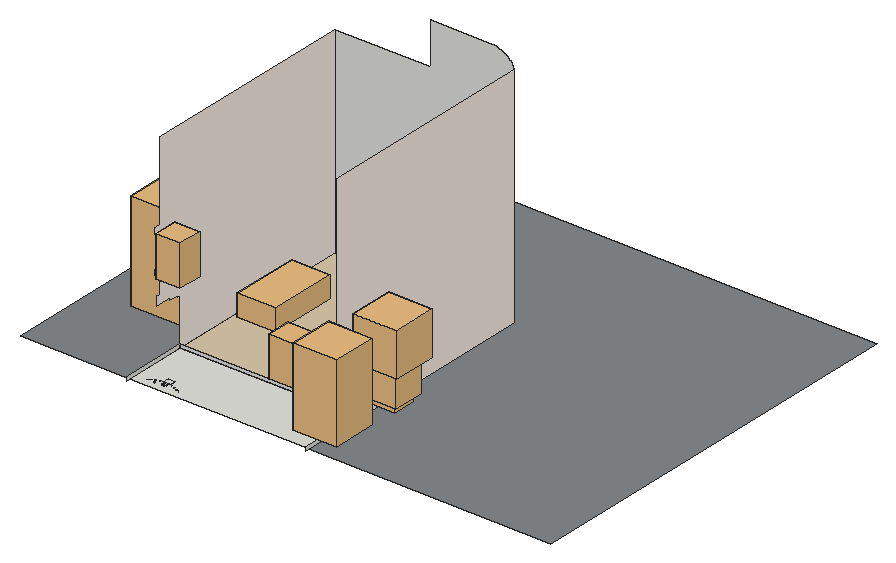
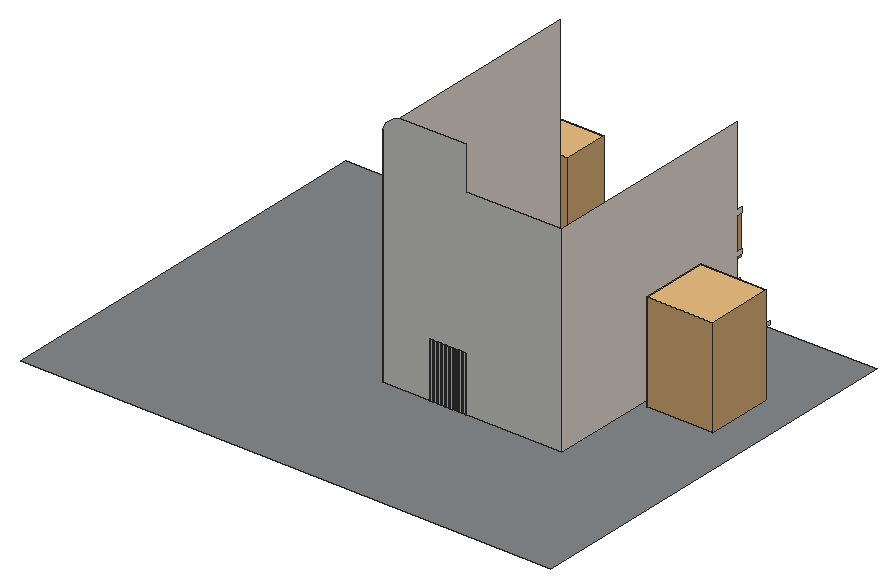
# SketchUp Ruby script. Lengths in inches.
U = 1.inch
M = Sketchup.active_model
def pt(a) = Geom::Point3d.new(a.map { |v| v * U })
def face(e, loops, mat)
  f = e.add_face(loops[0].map { |a| pt(a) })
  loops[1..].each { |l| e.add_face(l.map { |a| pt(a) }).erase! }
  f.material = f.back_material = mat if mat
  f
end
# faces: each face lists its corners as indices into pts; further lists are holes
def faces(e, pts, list, mat = nil) = list.each { |f| face(e, (f[0].is_a?(Array) ? f : [f]).map { |l| l.map { |i| pts[i] } }, mat) }
# xy, xz, yz: faces in a plane at the given z, y or x. An outline is a flat list of corners, or four numbers for a rectangle; further outlines are holes
def ring(l) = l.size == 4 ? [[l[0], l[1]], [l[2], l[1]], [l[2], l[3]], [l[0], l[3]]] : l.each_slice(2).to_a
def flat(e, list, mat, &to3) = list.each { |f| face(e, (f[0].is_a?(Array) ? f : [f]).map { |l| ring(l).map { |u, v| to3.(u, v) } }, mat) }
def xy(e, z, list, mat = nil) = flat(e, list, mat) { |x, y| [x, y, z] }
def xz(e, y, list, mat = nil) = flat(e, list, mat) { |x, z| [x, y, z] }
def yz(e, x, list, mat = nil) = flat(e, list, mat) { |y, z| [x, y, z] }
def lines(e, pts, list) = list.each { |a, b| e.add_line(pt(pts[a]), pt(pts[b])) }
# prism: a flat outline (further loops are holes) pulled along v
def prism(e, loops, v, mat = nil)
  f = face(e, loops, mat); d = Geom::Vector3d.new(v.map { |x| x * U })
  f.pushpull(f.normal.samedirection?(d) ? d.length : -d.length)
end
def box(e, o, s, mat = nil) = prism(e, [[o, [o[0] + s[0], o[1], o[2]], [o[0] + s[0], o[1] + s[1], o[2]], [o[0], o[1] + s[1], o[2]]]], [0, 0, s[2]], mat)
def at(x, y, z, deg = 0) = Geom::Transformation.translation(pt([x, y, z])) * Geom::Transformation.rotation(ORIGIN, Z_AXIS, deg.degrees)
def axes(o, x, y, z) = Geom::Transformation.new([*x, 0, *y, 0, *z, 0, *pt(o).to_a, 1])
def part(name) = M.definitions.add(name)
# library, detail: a bought-in or finely detailed component or shape, given as its bounding box
def library(name, o, s) = part(name).tap { |d| box(d.entities, o, s) }
def detail(e, o, s) = box(e.add_group.entities, o, s)
def put(e, d, t, mat = nil) = e.add_instance(d, t).tap { |i| i.material = mat if mat }
def group(e, t, mat = nil) = e.add_group.tap { |g| g.transformation = t; g.material = mat if mat }.entities
root = M.entities
M.materials.add("Material__3").color = [91, 133, 74]
M.materials.add("Material__4").color = [174, 125, 66]
M.materials.add("[0009_Linen]").color = [250, 240, 230]
M.materials.add("[Asphalt_Stamped_Brick]").color = [149, 133, 134]
M.materials.add("[Blacktop Old 01]").color = [132, 136, 139]
M.materials.add("[Brick_Colored_Blue]").color = [144, 143, 146]
M.materials.add("[Field Square Tile]").color = [217, 201, 169]
M.materials.add("[Metal_Steel_Textured_White]").color = [191, 191, 191]
c1 = library("Group\#1",[-35.09,50.53,0.35],[65,65.01,78.63])
c2 = library("Group\#5",[-64.15,18.03,113.23],[126.13,128.06,125.3])
c3 = library("Group\#6",[-43.12,34.07,23.92],[89.16,89.66,208.68])
c4 = library("Group\#120",[0,0,0],[26.57,25.63,42.93])
c5 = library("Group\#10",[-45.81,-5.78,22.29],[23.07,17.06,86])
c6 = library("Group\#3",[0,0,0],[46.67,47.38,83.02])
c7 = part("BAMBOO+PLANTS+18")
p = [[0,0,0],[1,0,0],[1,1,0]]
lines(c7.entities,p,[[0,1],[1,2],[2,0]])
put(c7.entities,c1,at(0,0,0))
put(c7.entities,c2,at(0,0,0),"Material__3")
put(c7.entities,c3,at(0,0,0),"Material__4")
put(c7.entities,c4,axes([-354.27,77.73,-57.76],[2.7027,0,0],[0,2.7027,0],[0,0,2.7027]))
put(c7.entities,c4,axes([-609.51,-13.32,151.65],[2.7027,0,0],[0,2.7027,0],[0,0,2.7027]))
put(c7.entities,c5,at(0,0,0),"Material__4")
put(c7.entities,c6,axes([-100.4,-152.87,0.24],[2.7027,0,0],[0,2.7027,0],[0,0,2.7027]))
put(c7.entities,c6,axes([-818.61,158.75,-120.63],[4.05405,0,0],[0,4.05405,0],[0,0,4.05405]))
c8 = library("office",[0,0,0],[107.02,69.62,36.57])
c9 = part("Vertical timber slat")
box(c9.entities,[0,0,0],[1.85,1.85,112.2])
c10 = part("Timber slat screen")
put(c10.entities,c9,at(0,0,0))
put(c10.entities,c9,at(0,13.1875,0))
put(c10.entities,c9,at(0,18.46,0))
put(c10.entities,c9,at(0,10.55,0))
put(c10.entities,c9,at(0,2.64,0))
put(c10.entities,c9,at(0,7.91,0))
put(c10.entities,c9,at(0,5.28,0))
put(c10.entities,c9,at(0,15.83,0))
put(c10.entities,c9,at(0,21.1,0))
xy(root,0,[[116.615,181.5,303.95,249.09],[303.95,181.5,308.325,249.09]])
xy(root,0,[[0,181.5,0,616,566.5625,616,566.5625,181.5,308.325,181.5,308.325,455.527,116.615,455.527,116.615,181.5]],"[Blacktop Old 01]")
xy(root,0,[[116.615,249.09,308.325,455.527]],"[Field Square Tile]")
xy(root,3.625,[[141.398,184.727,141.393,184.728,141.388,184.73,141.384,184.733,141.381,184.737,141.379,184.742,141.378,184.747,141.379,184.752,141.381,184.757,141.384,184.761,141.388,184.765,141.393,184.767,141.404,184.767,141.408,184.765,141.416,184.757,141.418,184.752,141.418,184.742,141.416,184.737,141.412,184.733,141.408,184.73,141.404,184.728],[148.82,185.161,148.815,185.162,148.81,185.164,148.806,185.167,148.803,185.171,148.801,185.176,148.8,185.181,148.801,185.187,148.803,185.191,148.806,185.196,148.81,185.199,148.815,185.201,148.825,185.201,148.83,185.199,148.834,185.196,148.837,185.191,148.839,185.187,148.84,185.181,148.839,185.176,148.837,185.171,148.834,185.167,148.83,185.164,148.825,185.162],[150.816,185.161,150.811,185.162,150.806,185.164,150.802,185.167,150.799,185.171,150.797,185.176,150.796,185.181,150.797,185.187,150.799,185.191,150.802,185.196,150.806,185.199,150.811,185.201,150.821,185.201,150.826,185.199,150.83,185.196,150.833,185.191,150.835,185.187,150.836,185.181,150.835,185.176,150.833,185.171,150.83,185.167,150.826,185.164,150.821,185.162],[163.155,185.926,163.15,185.927,163.145,185.929,163.141,185.932,163.138,185.936,163.136,185.941,163.135,185.946,163.136,185.951,163.138,185.956,163.141,185.96,163.145,185.964,163.15,185.966,163.161,185.966,163.165,185.964,163.173,185.956,163.175,185.951,163.175,185.941,163.173,185.936,163.169,185.932,163.165,185.929,163.161,185.927],[147.357,186.909,147.351,186.91,147.347,186.912,147.343,186.915,147.339,186.919,147.337,186.924,147.337,186.934,147.339,186.939,147.343,186.943,147.347,186.946,147.351,186.948,147.357,186.949,147.362,186.948,147.367,186.946,147.371,186.943,147.374,186.939,147.376,186.934,147.377,186.929,147.376,186.924,147.374,186.919,147.371,186.915,147.367,186.912,147.362,186.91],
  [152.279,186.909,152.274,186.91,152.269,186.912,152.265,186.915,152.262,186.919,152.26,186.924,152.259,186.929,152.26,186.934,152.262,186.939,152.265,186.943,152.269,186.946,152.274,186.948,152.279,186.949,152.284,186.948,152.289,186.946,152.293,186.943,152.296,186.939,152.298,186.934,152.299,186.929,152.298,186.924,152.296,186.919,152.293,186.915,152.289,186.912,152.284,186.91],[139.413,187.422,139.408,187.424,139.404,187.428,139.401,187.432,139.399,187.436,139.398,187.442,139.399,187.447,139.401,187.452,139.404,187.456,139.408,187.459,139.413,187.461,139.418,187.462,139.423,187.461,139.428,187.459,139.432,187.456,139.435,187.452,139.4375,187.447,139.438,187.442,139.4375,187.436,139.435,187.432,139.432,187.428,139.428,187.424,139.423,187.422],[140.156,187.727,140.151,187.728,140.146,187.73,140.142,187.733,140.138,187.737,140.136,187.742,140.136,187.752,140.138,187.757,140.142,187.761,140.146,187.764,140.151,187.766,140.156,187.767,140.161,187.766,140.166,187.764,140.17,187.761,140.173,187.757,140.175,187.752,140.176,187.747,140.175,187.742,140.173,187.737,140.17,187.733,140.166,187.73,140.161,187.728],[159.48,187.727,159.475,187.728,159.47,187.73,159.466,187.733,159.463,187.737,159.461,187.742,159.46,187.747,159.461,187.752,159.463,187.757,159.466,187.761,159.47,187.764,159.475,187.766,159.48,187.767,159.485,187.766,159.49,187.764,159.494,187.761,159.497,187.757,159.499,187.752,159.5,187.747,159.499,187.742,159.497,187.737,159.494,187.733,159.49,187.73,159.485,187.728],[156.044,188.822,156.039,188.824,156.035,188.827,156.032,188.831,156.03,188.836,156.029,188.841,156.03,188.847,156.032,188.851,156.035,188.856,156.039,188.859,156.044,188.861,156.054,188.861,156.059,188.859,156.063,188.856,156.066,188.851,156.068,188.847,156.069,188.841,156.068,188.836,156.066,188.831,156.063,188.827,156.059,188.824,156.054,188.822],
  [147.136,189.435,147.13,189.436,147.126,189.438,147.122,189.441,147.118,189.445,147.116,189.45,147.116,189.46,147.118,189.465,147.122,189.469,147.126,189.472,147.13,189.474,147.136,189.475,147.141,189.474,147.146,189.472,147.15,189.469,147.153,189.465,147.155,189.46,147.156,189.455,147.155,189.45,147.153,189.445,147.15,189.441,147.146,189.438,147.141,189.436],[148.537,189.542,148.532,189.544,148.528,189.548,148.525,189.552,148.523,189.557,148.522,189.562,148.523,189.567,148.525,189.572,148.528,189.576,148.532,189.579,148.537,189.581,148.542,189.582,148.547,189.581,148.552,189.579,148.556,189.576,148.56,189.572,148.562,189.567,148.562,189.557,148.56,189.552,148.552,189.544,148.547,189.542],[151.088,189.542,151.084,189.544,151.079,189.548,151.076,189.552,151.074,189.557,151.074,189.567,151.076,189.572,151.079,189.576,151.084,189.579,151.088,189.581,151.094,189.582,151.099,189.581,151.103,189.579,151.108,189.576,151.111,189.572,151.113,189.567,151.113,189.557,151.111,189.552,151.108,189.548,151.103,189.544,151.099,189.542]],"[Asphalt_Stamped_Brick]")
xy(root,3.625,[[148.272,184.789,148.267,184.793,148.262,184.796,148.258,184.799,148.238,184.811,148.233,184.815,148.234,184.82,148.234,184.832,148.235,184.838,148.235,184.849,148.236,184.855,148.236,184.861,148.241,184.863,148.246,184.866,148.251,184.868,148.256,184.871,148.262,184.874,148.267,184.876,148.272,184.879,148.277,184.881,148.292,184.872,148.296,184.869,148.306,184.863,148.311,184.859,148.316,184.856,148.315,184.85,148.315,184.839,148.314,184.833,148.314,184.822,148.313,184.816,148.313,184.81,148.308,184.808,148.298,184.802,148.293,184.8,148.287,184.797,148.282,184.795]],"[Brick_Colored_Blue]")
xy(root,3.625,[[[140.661,184.353,140.638,184.356,140.616,184.365,140.598,184.379,140.584,184.397,140.575,184.419,140.572,184.442,140.575,184.465,140.584,184.486,140.598,184.505,140.616,184.519,140.638,184.528,140.661,184.531,140.684,184.528,140.705,184.519,140.724,184.505,140.738,184.486,140.747,184.465,140.75,184.442,140.747,184.419,140.738,184.397,140.724,184.379,140.705,184.365,140.684,184.356],[140.661,184.354,140.683,184.357,140.705,184.366,140.723,184.38,140.737,184.398,140.746,184.419,140.749,184.442,140.746,184.464,140.737,184.486,140.723,184.504,140.705,184.518,140.683,184.527,140.661,184.53,140.638,184.527,140.617,184.518,140.599,184.504,140.585,184.486,140.576,184.464,140.573,184.442,140.576,184.419,140.585,184.398,140.599,184.38,140.617,184.366,140.638,184.357]],[[140.661,184.354,140.638,184.357,140.617,184.366,140.599,184.38,140.585,184.398,140.576,184.419,140.573,184.442,140.576,184.464,140.585,184.486,140.599,184.504,140.617,184.518,140.638,184.527,140.661,184.53,140.683,184.527,140.705,184.518,140.723,184.504,140.737,184.486,140.746,184.464,140.749,184.442,140.746,184.419,140.737,184.398,140.723,184.38,140.705,184.366,140.683,184.357],[140.661,184.405,140.67,184.406,140.679,184.41,140.687,184.416,140.692,184.423,140.696,184.432,140.697,184.442,140.696,184.451,140.692,184.46,140.687,184.468,140.679,184.473,140.67,184.477,140.661,184.478,140.651,184.477,140.642,184.473,140.635,184.468,140.629,184.46,140.625,184.451,140.624,184.442,140.625,184.432,140.629,184.423,140.635,184.416,140.642,184.41,140.651,184.406]],[[141.398,184.658,141.375,184.661,141.354,184.67,141.335,184.684,141.321,184.703,141.3125,184.724,141.309,184.747,141.3125,184.77,141.321,184.792,141.335,184.81,141.354,184.824,141.375,184.833,141.398,184.836,141.421,184.833,141.443,184.824,141.461,184.81,141.475,184.792,141.484,184.77,141.487,184.747,141.484,184.724,141.475,184.703,141.461,184.684,141.443,184.67,141.421,184.661],[141.398,184.659,141.421,184.662,141.442,184.671,141.461,184.685,141.474,184.703,141.483,184.724,141.486,184.747,141.483,184.77,141.474,184.791,141.461,184.809,141.442,184.823,141.421,184.832,141.398,184.835,141.376,184.832,141.354,184.823,141.336,184.809,141.322,184.791,141.313,184.77,141.31,184.747,141.313,184.724,141.322,184.703,141.336,184.685,141.354,184.671,141.376,184.662]],[[158.237,184.659,158.215,184.662,158.193,184.671,158.175,184.685,158.161,184.703,158.153,184.724,158.15,184.747,158.153,184.77,158.161,184.791,158.175,184.809,158.193,184.823,158.215,184.832,158.237,184.835,158.26,184.832,158.281,184.823,158.3,184.809,158.314,184.791,158.322,184.77,158.325,184.747,158.322,184.724,158.314,184.703,158.3,184.685,158.281,184.671,158.26,184.662],[158.237,184.711,158.247,184.712,158.256,184.716,158.263,184.721,158.269,184.729,158.273,184.738,158.274,184.747,158.273,184.757,158.269,184.766,158.263,184.773,158.256,184.779,158.247,184.783,158.237,184.784,158.228,184.783,158.219,184.779,158.212,184.773,158.206,184.766,158.202,184.757,158.201,184.747,158.202,184.738,158.206,184.729,158.212,184.721,158.219,184.716,158.228,184.712]],[[148.275,184.669,148.231,184.675,148.191,184.691,148.157,184.718,148.13,184.752,148.114,184.792,148.108,184.835,148.114,184.878,148.13,184.919,148.157,184.953,148.191,184.979,148.231,184.996,148.275,185.002,148.318,184.996,148.358,184.979,148.392,184.953,148.419,184.919,148.435,184.878,148.441,184.835,148.435,184.792,148.419,184.752,148.392,184.718,148.358,184.691,148.318,184.675],[148.275,184.716,148.306,184.72,148.334,184.732,148.359,184.751,148.378,184.776,148.39,184.804,148.394,184.835,148.39,184.866,148.378,184.895,148.359,184.92,148.334,184.939,148.306,184.951,148.275,184.955,148.244,184.951,148.215,184.939,148.19,184.92,148.171,184.895,148.159,184.866,148.155,184.835,148.159,184.804,148.171,184.776,148.19,184.751,148.215,184.732,148.244,184.72]],
  [[141.398,184.711,141.389,184.712,141.38,184.716,141.372,184.721,141.367,184.729,141.363,184.738,141.362,184.747,141.363,184.757,141.367,184.766,141.372,184.773,141.38,184.779,141.389,184.783,141.398,184.784,141.408,184.783,141.417,184.779,141.424,184.773,141.43,184.766,141.434,184.757,141.435,184.747,141.434,184.738,141.43,184.729,141.424,184.721,141.417,184.716,141.408,184.712],[141.398,184.727,141.404,184.728,141.408,184.73,141.412,184.733,141.416,184.737,141.418,184.742,141.418,184.752,141.416,184.757,141.408,184.765,141.404,184.767,141.393,184.767,141.388,184.765,141.384,184.761,141.381,184.757,141.379,184.752,141.378,184.747,141.379,184.742,141.381,184.737,141.384,184.733,141.388,184.73,141.393,184.728]],[[148.275,184.716,148.244,184.72,148.215,184.732,148.19,184.751,148.171,184.776,148.159,184.804,148.155,184.835,148.159,184.866,148.171,184.895,148.19,184.92,148.215,184.939,148.244,184.951,148.275,184.955,148.306,184.951,148.334,184.939,148.359,184.92,148.378,184.895,148.39,184.866,148.394,184.835,148.39,184.804,148.378,184.776,148.359,184.751,148.334,184.732,148.306,184.72],[148.272,184.789,148.282,184.795,148.287,184.797,148.293,184.8,148.298,184.802,148.308,184.808,148.313,184.81,148.313,184.816,148.314,184.822,148.314,184.833,148.315,184.839,148.315,184.85,148.316,184.856,148.311,184.859,148.306,184.863,148.296,184.869,148.292,184.872,148.277,184.881,148.272,184.879,148.267,184.876,148.262,184.874,148.256,184.871,148.251,184.868,148.246,184.866,148.241,184.863,148.236,184.861,148.236,184.855,148.235,184.849,148.235,184.838,148.234,184.832,148.234,184.82,148.233,184.815,148.238,184.811,148.258,184.799,148.262,184.796,148.267,184.793]],[[151.361,184.716,151.33,184.72,151.301,184.732,151.277,184.751,151.258,184.776,151.246,184.804,151.242,184.835,151.246,184.866,151.258,184.895,151.277,184.92,151.301,184.939,151.33,184.951,151.361,184.955,151.392,184.951,151.421,184.939,151.446,184.92,151.465,184.895,151.477,184.866,151.481,184.835,151.477,184.804,151.465,184.776,151.446,184.751,151.421,184.732,151.392,184.72],[151.359,184.789,151.369,184.795,151.374,184.797,151.379,184.8,151.384,184.802,151.39,184.805,151.395,184.808,151.4,184.81,151.4,184.822,151.401,184.827,151.401,184.839,151.402,184.845,151.402,184.856,151.398,184.859,151.393,184.863,151.373,184.875,151.369,184.878,151.364,184.881,151.359,184.879,151.354,184.876,151.348,184.874,151.338,184.868,151.333,184.866,151.328,184.863,151.323,184.861,151.322,184.855,151.322,184.843,151.321,184.838,151.321,184.826,151.32,184.82,151.32,184.815,151.325,184.811,151.335,184.805,151.339,184.802,151.354,184.793]],[151.359,184.789,151.354,184.793,151.339,184.802,151.335,184.805,151.325,184.811,151.32,184.815,151.32,184.82,151.321,184.826,151.321,184.838,151.322,184.843,151.322,184.855,151.323,184.861,151.328,184.863,151.333,184.866,151.338,184.868,151.348,184.874,151.354,184.876,151.359,184.879,151.364,184.881,151.369,184.878,151.373,184.875,151.393,184.863,151.398,184.859,151.402,184.856,151.402,184.845,151.401,184.839,151.401,184.827,151.4,184.822,151.4,184.81,151.395,184.808,151.39,184.805,151.384,184.802,151.379,184.8,151.374,184.797,151.369,184.795],[[148.82,185.093,148.797,185.096,148.775,185.104,148.757,185.119,148.743,185.137,148.734,185.158,148.731,185.181,148.734,185.204,148.743,185.226,148.757,185.244,148.775,185.258,148.797,185.267,148.82,185.27,148.843,185.267,148.864,185.258,148.883,185.244,148.897,185.226,148.906,185.204,148.909,185.181,148.906,185.158,148.897,185.137,148.883,185.119,148.864,185.104,148.843,185.096],[148.82,185.093,148.843,185.096,148.864,185.105,148.882,185.119,148.896,185.137,148.905,185.159,148.908,185.181,148.905,185.204,148.896,185.225,148.882,185.244,148.864,185.258,148.843,185.266,148.82,185.269,148.797,185.266,148.776,185.258,148.758,185.244,148.744,185.225,148.735,185.204,148.732,185.181,148.735,185.159,148.744,185.137,148.758,185.119,148.776,185.105,148.797,185.096]],
  [[150.816,185.093,150.793,185.096,150.771,185.104,150.753,185.119,150.739,185.137,150.73,185.158,150.727,185.181,150.73,185.204,150.739,185.226,150.753,185.244,150.771,185.258,150.793,185.267,150.816,185.27,150.839,185.267,150.86,185.258,150.879,185.244,150.893,185.226,150.902,185.204,150.905,185.181,150.902,185.158,150.893,185.137,150.879,185.119,150.86,185.104,150.839,185.096],[150.816,185.093,150.839,185.096,150.86,185.105,150.878,185.119,150.892,185.137,150.901,185.159,150.904,185.181,150.901,185.204,150.892,185.225,150.878,185.244,150.86,185.258,150.839,185.266,150.816,185.269,150.793,185.266,150.772,185.258,150.754,185.244,150.74,185.225,150.731,185.204,150.728,185.181,150.731,185.159,150.74,185.137,150.754,185.119,150.772,185.105,150.793,185.096]],[149.818,185.128,149.804,185.13,149.791,185.135,149.78,185.144,149.772,185.155,149.766,185.168,149.765,185.181,149.766,185.195,149.772,185.208,149.78,185.219,149.791,185.227,149.804,185.233,149.818,185.235],[149.818,185.128,149.818,185.235,149.832,185.233,149.845,185.227,149.856,185.219,149.864,185.208,149.869,185.195,149.871,185.181,149.869,185.168,149.864,185.155,149.856,185.144,149.845,185.135,149.832,185.13],[[148.82,185.145,148.81,185.146,148.802,185.15,148.794,185.156,148.788,185.163,148.784,185.172,148.783,185.181,148.784,185.191,148.788,185.2,148.794,185.207,148.802,185.213,148.81,185.217,148.82,185.218,148.829,185.217,148.838,185.213,148.846,185.207,148.852,185.2,148.855,185.191,148.856,185.181,148.855,185.172,148.852,185.163,148.846,185.156,148.838,185.15,148.829,185.146],[148.82,185.161,148.825,185.162,148.83,185.164,148.834,185.167,148.837,185.171,148.839,185.176,148.84,185.181,148.839,185.187,148.837,185.191,148.834,185.196,148.83,185.199,148.825,185.201,148.815,185.201,148.81,185.199,148.806,185.196,148.803,185.191,148.801,185.187,148.8,185.181,148.801,185.176,148.803,185.171,148.806,185.167,148.81,185.164,148.815,185.162]],[[150.816,185.145,150.806,185.146,150.798,185.15,150.79,185.156,150.784,185.163,150.781,185.172,150.779,185.181,150.781,185.191,150.784,185.2,150.79,185.207,150.798,185.213,150.806,185.217,150.816,185.218,150.825,185.217,150.834,185.213,150.842,185.207,150.848,185.2,150.851,185.191,150.853,185.181,150.851,185.172,150.848,185.163,150.842,185.156,150.834,185.15,150.825,185.146],[150.816,185.161,150.821,185.162,150.826,185.164,150.83,185.167,150.833,185.171,150.835,185.176,150.836,185.181,150.835,185.187,150.833,185.191,150.83,185.196,150.826,185.199,150.821,185.201,150.811,185.201,150.806,185.199,150.802,185.196,150.799,185.191,150.797,185.187,150.796,185.181,150.797,185.176,150.799,185.171,150.802,185.167,150.806,185.164,150.811,185.162]],
  [[136.48,185.857,136.457,185.86,136.436,185.869,136.418,185.883,136.403,185.902,136.395,185.923,136.392,185.946,136.395,185.969,136.403,185.991,136.418,186.009,136.436,186.023,136.457,186.032,136.48,186.035,136.503,186.032,136.525,186.023,136.543,186.009,136.557,185.991,136.566,185.969,136.569,185.946,136.566,185.923,136.557,185.902,136.543,185.883,136.525,185.869,136.503,185.86],[136.48,185.858,136.503,185.861,136.524,185.87,136.543,185.884,136.557,185.902,136.565,185.924,136.568,185.946,136.565,185.969,136.557,185.99,136.543,186.008,136.524,186.022,136.503,186.031,136.48,186.034,136.458,186.031,136.436,186.022,136.418,186.008,136.404,185.99,136.395,185.969,136.392,185.946,136.395,185.924,136.404,185.902,136.418,185.884,136.436,185.87,136.458,185.861]],[[163.155,185.857,163.132,185.86,163.111,185.869,163.093,185.883,163.078,185.902,163.07,185.923,163.066,185.946,163.07,185.969,163.078,185.991,163.093,186.009,163.111,186.023,163.132,186.032,163.155,186.035,163.178,186.032,163.2,186.023,163.218,186.009,163.232,185.991,163.241,185.969,163.244,185.946,163.241,185.923,163.232,185.902,163.218,185.883,163.2,185.869,163.178,185.86],[163.155,185.858,163.178,185.861,163.199,185.87,163.218,185.884,163.232,185.902,163.24,185.924,163.243,185.946,163.24,185.969,163.232,185.99,163.218,186.008,163.199,186.022,163.178,186.031,163.155,186.034,163.133,186.031,163.111,186.022,163.093,186.008,163.079,185.99,163.07,185.969,163.067,185.946,163.07,185.924,163.079,185.902,163.093,185.884,163.111,185.87,163.133,185.861]],[[163.155,185.858,163.133,185.861,163.111,185.87,163.093,185.884,163.079,185.902,163.07,185.924,163.067,185.946,163.07,185.969,163.079,185.99,163.093,186.008,163.111,186.022,163.133,186.031,163.155,186.034,163.178,186.031,163.199,186.022,163.218,186.008,163.232,185.99,163.24,185.969,163.243,185.946,163.24,185.924,163.232,185.902,163.218,185.884,163.199,185.87,163.178,185.861],[163.155,185.91,163.165,185.911,163.174,185.915,163.181,185.92,163.187,185.928,163.191,185.937,163.192,185.946,163.191,185.956,163.187,185.965,163.181,185.972,163.174,185.978,163.165,185.982,163.155,185.983,163.146,185.982,163.137,185.978,163.13,185.972,163.124,185.965,163.12,185.956,163.119,185.946,163.12,185.937,163.124,185.928,163.13,185.92,163.137,185.915,163.146,185.911]],[[163.155,185.91,163.146,185.911,163.137,185.915,163.13,185.92,163.124,185.928,163.12,185.937,163.119,185.946,163.12,185.956,163.124,185.965,163.13,185.972,163.137,185.978,163.146,185.982,163.155,185.983,163.165,185.982,163.174,185.978,163.181,185.972,163.187,185.965,163.191,185.956,163.192,185.946,163.191,185.937,163.187,185.928,163.181,185.92,163.174,185.915,163.165,185.911],[163.155,185.926,163.161,185.927,163.165,185.929,163.169,185.932,163.173,185.936,163.175,185.941,163.175,185.951,163.173,185.956,163.165,185.964,163.161,185.966,163.15,185.966,163.145,185.964,163.141,185.96,163.138,185.956,163.136,185.951,163.135,185.946,163.136,185.941,163.138,185.936,163.141,185.932,163.145,185.929,163.15,185.927]],[[147.357,186.84,147.334,186.843,147.312,186.852,147.294,186.866,147.28,186.885,147.271,186.906,147.268,186.929,147.271,186.952,147.28,186.973,147.294,186.992,147.312,187.006,147.334,187.015,147.357,187.018,147.38,187.015,147.401,187.006,147.42,186.992,147.434,186.973,147.443,186.952,147.446,186.929,147.443,186.906,147.434,186.885,147.42,186.866,147.401,186.852,147.38,186.843],[147.357,186.841,147.379,186.844,147.401,186.853,147.419,186.867,147.433,186.885,147.442,186.906,147.445,186.929,147.442,186.952,147.433,186.973,147.419,186.991,147.401,187.005,147.379,187.014,147.357,187.017,147.334,187.014,147.3125,187.005,147.294,186.991,147.281,186.973,147.272,186.952,147.269,186.929,147.272,186.906,147.281,186.885,147.294,186.867,147.3125,186.853,147.334,186.844]],
  [[152.279,186.84,152.256,186.843,152.235,186.852,152.216,186.866,152.202,186.885,152.193,186.906,152.19,186.929,152.193,186.952,152.202,186.973,152.216,186.992,152.235,187.006,152.256,187.015,152.279,187.018,152.302,187.015,152.324,187.006,152.342,186.992,152.356,186.973,152.365,186.952,152.368,186.929,152.365,186.906,152.356,186.885,152.342,186.866,152.324,186.852,152.302,186.843],[152.279,186.841,152.302,186.844,152.323,186.853,152.341,186.867,152.355,186.885,152.364,186.906,152.367,186.929,152.364,186.952,152.355,186.973,152.341,186.991,152.323,187.005,152.302,187.014,152.279,187.017,152.256,187.014,152.235,187.005,152.217,186.991,152.203,186.973,152.194,186.952,152.191,186.929,152.194,186.906,152.203,186.885,152.217,186.867,152.235,186.853,152.256,186.844]],[[147.357,186.892,147.347,186.894,147.338,186.897,147.331,186.903,147.325,186.911,147.321,186.92,147.32,186.929,147.321,186.939,147.325,186.947,147.331,186.955,147.338,186.961,147.347,186.964,147.357,186.966,147.366,186.964,147.375,186.961,147.383,186.955,147.388,186.947,147.392,186.939,147.393,186.929,147.392,186.92,147.388,186.911,147.383,186.903,147.375,186.897,147.366,186.894],[147.357,186.909,147.362,186.91,147.367,186.912,147.371,186.915,147.374,186.919,147.376,186.924,147.377,186.929,147.376,186.934,147.374,186.939,147.371,186.943,147.367,186.946,147.362,186.948,147.357,186.949,147.351,186.948,147.347,186.946,147.343,186.943,147.339,186.939,147.337,186.934,147.337,186.924,147.339,186.919,147.343,186.915,147.347,186.912,147.351,186.91]],[[152.279,186.892,152.27,186.894,152.261,186.897,152.253,186.903,152.247,186.911,152.244,186.92,152.243,186.929,152.244,186.939,152.247,186.947,152.253,186.955,152.261,186.961,152.27,186.964,152.279,186.966,152.289,186.964,152.297,186.961,152.305,186.955,152.311,186.947,152.314,186.939,152.316,186.929,152.314,186.92,152.311,186.911,152.305,186.903,152.297,186.897,152.289,186.894],[152.279,186.909,152.284,186.91,152.289,186.912,152.293,186.915,152.296,186.919,152.298,186.924,152.299,186.929,152.298,186.934,152.296,186.939,152.293,186.943,152.289,186.946,152.284,186.948,152.279,186.949,152.274,186.948,152.269,186.946,152.265,186.943,152.262,186.939,152.26,186.934,152.259,186.929,152.26,186.924,152.262,186.919,152.265,186.915,152.269,186.912,152.274,186.91]],[[139.418,187.353,139.395,187.356,139.374,187.365,139.355,187.379,139.341,187.397,139.332,187.419,139.329,187.442,139.332,187.465,139.341,187.486,139.355,187.505,139.374,187.519,139.395,187.528,139.418,187.531,139.441,187.528,139.462,187.519,139.481,187.505,139.495,187.486,139.504,187.465,139.507,187.442,139.504,187.419,139.495,187.397,139.481,187.379,139.462,187.365,139.441,187.356],[139.418,187.354,139.441,187.357,139.462,187.366,139.48,187.379,139.494,187.398,139.503,187.419,139.506,187.442,139.503,187.464,139.494,187.486,139.48,187.504,139.462,187.518,139.441,187.527,139.418,187.53,139.395,187.527,139.374,187.518,139.356,187.504,139.342,187.486,139.333,187.464,139.33,187.442,139.333,187.419,139.342,187.398,139.356,187.379,139.374,187.366,139.395,187.357]],[[139.418,187.354,139.395,187.357,139.374,187.366,139.356,187.379,139.342,187.398,139.333,187.419,139.33,187.442,139.333,187.464,139.342,187.486,139.356,187.504,139.374,187.518,139.395,187.527,139.418,187.53,139.441,187.527,139.462,187.518,139.48,187.504,139.494,187.486,139.503,187.464,139.506,187.442,139.503,187.419,139.494,187.398,139.48,187.379,139.462,187.366,139.441,187.357],[139.418,187.405,139.428,187.406,139.436,187.41,139.444,187.416,139.45,187.423,139.453,187.432,139.455,187.442,139.453,187.451,139.45,187.46,139.444,187.468,139.436,187.473,139.428,187.477,139.418,187.478,139.409,187.477,139.4,187.473,139.392,187.468,139.386,187.46,139.383,187.451,139.381,187.442,139.383,187.432,139.386,187.423,139.392,187.416,139.4,187.41,139.409,187.406]],
  [[160.218,187.354,160.195,187.357,160.174,187.366,160.156,187.379,160.142,187.398,160.133,187.419,160.13,187.442,160.133,187.464,160.142,187.486,160.156,187.504,160.174,187.518,160.195,187.527,160.218,187.53,160.24,187.527,160.262,187.518,160.28,187.504,160.294,187.486,160.303,187.464,160.306,187.442,160.303,187.419,160.294,187.398,160.28,187.379,160.262,187.366,160.24,187.357],[160.218,187.405,160.227,187.406,160.236,187.41,160.244,187.416,160.249,187.423,160.253,187.432,160.254,187.442,160.253,187.451,160.249,187.46,160.244,187.468,160.236,187.473,160.227,187.477,160.218,187.478,160.208,187.477,160.199,187.473,160.192,187.468,160.186,187.46,160.182,187.451,160.181,187.442,160.182,187.432,160.186,187.423,160.192,187.416,160.199,187.41,160.208,187.406]],[[139.418,187.405,139.409,187.406,139.4,187.41,139.392,187.416,139.386,187.423,139.383,187.432,139.381,187.442,139.383,187.451,139.386,187.46,139.392,187.468,139.4,187.473,139.409,187.477,139.418,187.478,139.428,187.477,139.436,187.473,139.444,187.468,139.45,187.46,139.453,187.451,139.455,187.442,139.453,187.432,139.45,187.423,139.444,187.416,139.436,187.41,139.428,187.406],[139.413,187.422,139.423,187.422,139.428,187.424,139.432,187.428,139.435,187.432,139.4375,187.436,139.438,187.442,139.4375,187.447,139.435,187.452,139.432,187.456,139.428,187.459,139.423,187.461,139.418,187.462,139.413,187.461,139.408,187.459,139.404,187.456,139.401,187.452,139.399,187.447,139.398,187.442,139.399,187.436,139.401,187.432,139.404,187.428,139.408,187.424]],[[160.218,187.405,160.208,187.406,160.199,187.41,160.192,187.416,160.186,187.423,160.182,187.432,160.181,187.442,160.182,187.451,160.186,187.46,160.192,187.468,160.199,187.473,160.208,187.477,160.218,187.478,160.227,187.477,160.236,187.473,160.244,187.468,160.249,187.46,160.253,187.451,160.254,187.442,160.253,187.432,160.249,187.423,160.244,187.416,160.236,187.41,160.227,187.406],[160.213,187.422,160.223,187.422,160.228,187.424,160.232,187.428,160.235,187.432,160.237,187.436,160.238,187.442,160.237,187.447,160.235,187.452,160.232,187.456,160.228,187.459,160.223,187.461,160.218,187.462,160.213,187.461,160.208,187.459,160.204,187.456,160.2,187.452,160.198,187.447,160.198,187.436,160.2,187.432,160.208,187.424]],[[159.48,187.658,159.457,187.661,159.436,187.67,159.417,187.684,159.403,187.703,159.394,187.724,159.391,187.747,159.394,187.77,159.403,187.792,159.417,187.81,159.436,187.824,159.457,187.833,159.48,187.836,159.503,187.833,159.525,187.824,159.543,187.81,159.557,187.792,159.566,187.77,159.569,187.747,159.566,187.724,159.557,187.703,159.543,187.684,159.525,187.67,159.503,187.661],[159.48,187.659,159.503,187.662,159.524,187.671,159.542,187.685,159.556,187.703,159.565,187.724,159.568,187.747,159.565,187.77,159.556,187.791,159.542,187.809,159.524,187.823,159.503,187.832,159.48,187.835,159.457,187.832,159.436,187.823,159.418,187.809,159.404,187.791,159.395,187.77,159.392,187.747,159.395,187.724,159.404,187.703,159.418,187.685,159.436,187.671,159.457,187.662]],[[140.156,187.711,140.146,187.712,140.137,187.716,140.13,187.721,140.124,187.729,140.12,187.738,140.119,187.747,140.12,187.757,140.124,187.765,140.13,187.773,140.137,187.779,140.146,187.783,140.156,187.784,140.165,187.783,140.174,187.779,140.182,187.773,140.1875,187.765,140.191,187.757,140.192,187.747,140.191,187.738,140.1875,187.729,140.182,187.721,140.174,187.716,140.165,187.712],[140.156,187.727,140.161,187.728,140.166,187.73,140.17,187.733,140.173,187.737,140.175,187.742,140.176,187.747,140.175,187.752,140.173,187.757,140.17,187.761,140.166,187.764,140.161,187.766,140.156,187.767,140.151,187.766,140.146,187.764,140.142,187.761,140.138,187.757,140.136,187.752,140.136,187.742,140.138,187.737,140.142,187.733,140.146,187.73,140.151,187.728]],
  [[159.48,187.711,159.471,187.712,159.462,187.716,159.454,187.721,159.448,187.729,159.445,187.738,159.443,187.747,159.445,187.757,159.448,187.765,159.454,187.773,159.462,187.779,159.471,187.783,159.48,187.784,159.49,187.783,159.498,187.779,159.506,187.773,159.512,187.765,159.515,187.757,159.517,187.747,159.515,187.738,159.512,187.729,159.506,187.721,159.498,187.716,159.49,187.712],[159.48,187.727,159.485,187.728,159.49,187.73,159.494,187.733,159.497,187.737,159.499,187.742,159.5,187.747,159.499,187.752,159.497,187.757,159.494,187.761,159.49,187.764,159.485,187.766,159.48,187.767,159.475,187.766,159.47,187.764,159.466,187.761,159.463,187.757,159.461,187.752,159.46,187.747,159.461,187.742,159.463,187.737,159.466,187.733,159.47,187.73,159.475,187.728]],[[147.992,187.895,147.949,187.901,147.909,187.917,147.875,187.944,147.848,187.978,147.832,188.018,147.826,188.062,147.832,188.105,147.848,188.145,147.875,188.179,147.909,188.206,147.949,188.222,147.992,188.228,148.035,188.222,148.075,188.206,148.11,188.179,148.136,188.145,148.153,188.105,148.159,188.062,148.153,188.018,148.136,187.978,148.11,187.944,148.075,187.917,148.035,187.901],[147.992,187.942,148.023,187.946,148.052,187.958,148.077,187.977,148.096,188.002,148.108,188.031,148.112,188.062,148.108,188.093,148.096,188.121,148.077,188.146,148.052,188.165,148.023,188.177,147.992,188.181,147.961,188.177,147.932,188.165,147.908,188.146,147.889,188.121,147.877,188.093,147.873,188.062,147.877,188.031,147.889,188.002,147.908,187.977,147.932,187.958,147.961,187.946]],[[151.644,187.895,151.6,187.901,151.56,187.917,151.526,187.944,151.499,187.978,151.483,188.018,151.477,188.062,151.483,188.105,151.499,188.145,151.526,188.179,151.56,188.206,151.6,188.222,151.644,188.228,151.687,188.222,151.727,188.206,151.761,188.179,151.788,188.145,151.804,188.105,151.81,188.062,151.804,188.018,151.788,187.978,151.761,187.944,151.727,187.917,151.687,187.901],[151.644,187.942,151.675,187.946,151.703,187.958,151.728,187.977,151.747,188.002,151.759,188.031,151.763,188.062,151.759,188.093,151.747,188.121,151.728,188.146,151.703,188.165,151.675,188.177,151.644,188.181,151.613,188.177,151.584,188.165,151.559,188.146,151.54,188.121,151.528,188.093,151.524,188.062,151.528,188.031,151.54,188.002,151.559,187.977,151.584,187.958,151.613,187.946]],[[147.992,187.942,147.961,187.946,147.932,187.958,147.908,187.977,147.889,188.002,147.877,188.031,147.873,188.062,147.877,188.093,147.889,188.121,147.908,188.146,147.932,188.165,147.961,188.177,147.992,188.181,148.023,188.177,148.052,188.165,148.077,188.146,148.096,188.121,148.108,188.093,148.112,188.062,148.108,188.031,148.096,188.002,148.077,187.977,148.052,187.958,148.023,187.946],[147.99,188.016,147.995,188.018,148,188.021,148.005,188.023,148.015,188.029,148.021,188.031,148.026,188.034,148.031,188.036,148.031,188.048,148.032,188.054,148.032,188.065,148.033,188.071,148.033,188.082,148.029,188.085,148.024,188.089,148.004,188.101,148,188.104,147.995,188.108,147.985,188.102,147.979,188.1,147.974,188.097,147.969,188.095,147.959,188.089,147.954,188.087,147.953,188.081,147.953,188.07,147.952,188.064,147.952,188.052,147.951,188.046,147.951,188.041,147.956,188.038,147.961,188.034,147.966,188.031,147.97,188.028]],[[151.644,187.942,151.613,187.946,151.584,187.958,151.559,187.977,151.54,188.002,151.528,188.031,151.524,188.062,151.528,188.093,151.54,188.121,151.559,188.146,151.584,188.165,151.613,188.177,151.644,188.181,151.675,188.177,151.703,188.165,151.728,188.146,151.747,188.121,151.759,188.093,151.763,188.062,151.759,188.031,151.747,188.002,151.728,187.977,151.703,187.958,151.675,187.946],[151.641,188.016,151.646,188.018,151.651,188.021,151.656,188.023,151.662,188.026,151.667,188.029,151.672,188.031,151.677,188.034,151.682,188.036,151.682,188.042,151.683,188.048,151.683,188.059,151.684,188.065,151.684,188.077,151.685,188.082,151.68,188.085,151.675,188.089,151.665,188.095,151.661,188.098,151.651,188.104,151.646,188.108,151.636,188.102,151.631,188.1,151.625,188.097,151.62,188.095,151.61,188.089,151.605,188.087,151.605,188.081,151.604,188.075,151.604,188.064,151.603,188.058,151.603,188.046,151.602,188.041,151.607,188.038,151.612,188.034,151.627,188.025,151.631,188.022]],
  [147.99,188.016,147.97,188.028,147.966,188.031,147.961,188.034,147.956,188.038,147.951,188.041,147.951,188.046,147.952,188.052,147.952,188.064,147.953,188.07,147.953,188.081,147.954,188.087,147.959,188.089,147.969,188.095,147.974,188.097,147.979,188.1,147.985,188.102,147.995,188.108,148,188.104,148.004,188.101,148.024,188.089,148.029,188.085,148.033,188.082,148.033,188.071,148.032,188.065,148.032,188.054,148.031,188.048,148.031,188.036,148.026,188.034,148.021,188.031,148.015,188.029,148.005,188.023,148,188.021,147.995,188.018],[151.641,188.016,151.631,188.022,151.627,188.025,151.612,188.034,151.607,188.038,151.602,188.041,151.603,188.046,151.603,188.058,151.604,188.064,151.604,188.075,151.605,188.081,151.605,188.087,151.61,188.089,151.62,188.095,151.625,188.097,151.631,188.1,151.636,188.102,151.646,188.108,151.651,188.104,151.661,188.098,151.665,188.095,151.675,188.089,151.68,188.085,151.685,188.082,151.684,188.077,151.684,188.065,151.683,188.059,151.683,188.048,151.682,188.042,151.682,188.036,151.677,188.034,151.672,188.031,151.667,188.029,151.662,188.026,151.656,188.023,151.651,188.021,151.646,188.018],[[143.587,188.754,143.564,188.757,143.543,188.765,143.525,188.779,143.511,188.798,143.502,188.819,143.499,188.841,143.502,188.864,143.511,188.885,143.525,188.904,143.543,188.918,143.564,188.926,143.587,188.929,143.61,188.926,143.631,188.918,143.649,188.904,143.663,188.885,143.672,188.864,143.675,188.841,143.672,188.819,143.663,188.798,143.649,188.779,143.631,188.765,143.61,188.757],[143.587,188.805,143.596,188.806,143.605,188.81,143.613,188.816,143.619,188.823,143.622,188.832,143.623,188.841,143.622,188.851,143.619,188.86,143.613,188.867,143.605,188.873,143.596,188.877,143.587,188.878,143.577,188.877,143.569,188.873,143.561,188.867,143.555,188.86,143.552,188.851,143.55,188.841,143.552,188.832,143.555,188.823,143.561,188.816,143.569,188.81,143.577,188.806]],[[156.049,188.754,156.026,188.757,156.005,188.765,155.987,188.779,155.973,188.798,155.964,188.819,155.961,188.841,155.964,188.864,155.973,188.885,155.987,188.904,156.005,188.918,156.026,188.926,156.049,188.929,156.072,188.926,156.093,188.918,156.111,188.904,156.125,188.885,156.134,188.864,156.137,188.841,156.134,188.819,156.125,188.798,156.111,188.779,156.093,188.765,156.072,188.757],[156.049,188.805,156.058,188.806,156.067,188.81,156.075,188.816,156.081,188.823,156.084,188.832,156.086,188.841,156.084,188.851,156.081,188.86,156.075,188.867,156.067,188.873,156.058,188.877,156.049,188.878,156.039,188.877,156.031,188.873,156.023,188.867,156.017,188.86,156.014,188.851,156.012,188.841,156.014,188.832,156.017,188.823,156.023,188.816,156.031,188.81,156.039,188.806]],[[156.049,188.805,156.039,188.806,156.031,188.81,156.023,188.816,156.017,188.823,156.014,188.832,156.012,188.841,156.014,188.851,156.017,188.86,156.023,188.867,156.031,188.873,156.039,188.877,156.049,188.878,156.058,188.877,156.067,188.873,156.075,188.867,156.081,188.86,156.084,188.851,156.086,188.841,156.084,188.832,156.081,188.823,156.075,188.816,156.067,188.81,156.058,188.806],[156.044,188.822,156.054,188.822,156.059,188.824,156.063,188.827,156.066,188.831,156.068,188.836,156.069,188.841,156.068,188.847,156.066,188.851,156.063,188.856,156.059,188.859,156.054,188.861,156.044,188.861,156.039,188.859,156.035,188.856,156.032,188.851,156.03,188.847,156.029,188.841,156.03,188.836,156.032,188.831,156.035,188.827,156.039,188.824]],
  [143.582,188.822,143.577,188.824,143.573,188.827,143.57,188.831,143.568,188.836,143.567,188.841,143.568,188.847,143.57,188.851,143.573,188.856,143.577,188.859,143.582,188.861,143.592,188.861,143.597,188.859,143.601,188.856,143.604,188.851,143.606,188.847,143.607,188.841,143.606,188.836,143.604,188.831,143.601,188.827,143.597,188.824,143.592,188.822],[[147.136,189.367,147.113,189.37,147.092,189.379,147.073,189.393,147.059,189.411,147.051,189.432,147.048,189.455,147.051,189.478,147.059,189.499,147.073,189.517,147.092,189.531,147.113,189.54,147.136,189.543,147.158,189.54,147.18,189.531,147.198,189.517,147.212,189.499,147.221,189.478,147.224,189.455,147.221,189.432,147.212,189.411,147.198,189.393,147.18,189.379,147.158,189.37],[147.136,189.419,147.145,189.42,147.154,189.423,147.162,189.429,147.167,189.437,147.171,189.446,147.172,189.455,147.171,189.465,147.167,189.473,147.162,189.481,147.154,189.487,147.145,189.491,147.136,189.492,147.126,189.491,147.117,189.487,147.11,189.481,147.104,189.473,147.1,189.465,147.099,189.455,147.1,189.446,147.104,189.437,147.11,189.429,147.117,189.423,147.126,189.42]],[[152.5,189.367,152.477,189.37,152.456,189.379,152.438,189.393,152.424,189.411,152.415,189.432,152.412,189.455,152.415,189.478,152.424,189.499,152.438,189.517,152.456,189.531,152.477,189.54,152.5,189.543,152.523,189.54,152.544,189.531,152.5625,189.517,152.576,189.499,152.585,189.478,152.588,189.455,152.585,189.432,152.576,189.411,152.5625,189.393,152.544,189.379,152.523,189.37],[152.5,189.419,152.51,189.42,152.518,189.423,152.526,189.429,152.532,189.437,152.535,189.446,152.537,189.455,152.535,189.465,152.532,189.473,152.526,189.481,152.518,189.487,152.51,189.491,152.5,189.492,152.491,189.491,152.482,189.487,152.474,189.481,152.468,189.473,152.465,189.465,152.464,189.455,152.465,189.446,152.468,189.437,152.474,189.429,152.482,189.423,152.491,189.42]],[[147.136,189.419,147.126,189.42,147.117,189.423,147.11,189.429,147.104,189.437,147.1,189.446,147.099,189.455,147.1,189.465,147.104,189.473,147.11,189.481,147.117,189.487,147.126,189.491,147.136,189.492,147.145,189.491,147.154,189.487,147.162,189.481,147.167,189.473,147.171,189.465,147.172,189.455,147.171,189.446,147.167,189.437,147.162,189.429,147.154,189.423,147.145,189.42],[147.136,189.435,147.141,189.436,147.146,189.438,147.15,189.441,147.153,189.445,147.155,189.45,147.156,189.455,147.155,189.46,147.153,189.465,147.15,189.469,147.146,189.472,147.141,189.474,147.136,189.475,147.13,189.474,147.126,189.472,147.122,189.469,147.118,189.465,147.116,189.46,147.116,189.45,147.118,189.445,147.122,189.441,147.126,189.438,147.13,189.436]],[[147.859,189.42,147.816,189.426,147.776,189.442,147.741,189.469,147.715,189.503,147.698,189.543,147.693,189.586,147.698,189.629,147.715,189.669,147.741,189.704,147.776,189.73,147.816,189.747,147.859,189.753,147.902,189.747,147.942,189.73,147.976,189.704,148.003,189.669,148.02,189.629,148.025,189.586,148.02,189.543,148.003,189.503,147.976,189.469,147.942,189.442,147.902,189.426],[147.859,189.466,147.89,189.47,147.919,189.482,147.944,189.501,147.963,189.526,147.975,189.555,147.979,189.586,147.975,189.617,147.963,189.646,147.944,189.671,147.919,189.69,147.89,189.702,147.859,189.706,147.828,189.702,147.799,189.69,147.774,189.671,147.755,189.646,147.743,189.617,147.739,189.586,147.743,189.555,147.755,189.526,147.774,189.501,147.799,189.482,147.828,189.47]],
  [[151.777,189.42,151.734,189.426,151.694,189.442,151.659,189.469,151.633,189.503,151.616,189.543,151.611,189.586,151.616,189.629,151.633,189.669,151.659,189.704,151.694,189.73,151.734,189.747,151.777,189.753,151.82,189.747,151.86,189.73,151.895,189.704,151.921,189.669,151.9375,189.629,151.943,189.586,151.9375,189.543,151.921,189.503,151.895,189.469,151.86,189.442,151.82,189.426],[151.777,189.466,151.808,189.47,151.837,189.482,151.862,189.501,151.881,189.526,151.893,189.555,151.897,189.586,151.893,189.617,151.881,189.646,151.862,189.671,151.837,189.69,151.808,189.702,151.777,189.706,151.746,189.702,151.717,189.69,151.692,189.671,151.673,189.646,151.661,189.617,151.657,189.586,151.661,189.555,151.673,189.526,151.692,189.501,151.717,189.482,151.746,189.47]],[[147.859,189.466,147.828,189.47,147.799,189.482,147.774,189.501,147.755,189.526,147.743,189.555,147.739,189.586,147.743,189.617,147.755,189.646,147.774,189.671,147.799,189.69,147.828,189.702,147.859,189.706,147.89,189.702,147.919,189.69,147.944,189.671,147.963,189.646,147.975,189.617,147.979,189.586,147.975,189.555,147.963,189.526,147.944,189.501,147.919,189.482,147.89,189.47],[147.856,189.54,147.861,189.543,147.867,189.545,147.877,189.551,147.882,189.553,147.887,189.556,147.892,189.558,147.897,189.561,147.898,189.567,147.898,189.578,147.899,189.584,147.899,189.596,147.9,189.601,147.9,189.607,147.89,189.613,147.886,189.616,147.881,189.62,147.861,189.632,147.856,189.63,147.846,189.624,147.841,189.622,147.836,189.619,147.831,189.617,147.825,189.614,147.82,189.611,147.82,189.6,147.819,189.594,147.819,189.583,147.818,189.577,147.818,189.565,147.823,189.562,147.827,189.559,147.842,189.55,147.847,189.546,147.852,189.543]],[[151.777,189.466,151.746,189.47,151.717,189.482,151.692,189.501,151.673,189.526,151.661,189.555,151.657,189.586,151.661,189.617,151.673,189.646,151.692,189.671,151.717,189.69,151.746,189.702,151.777,189.706,151.808,189.702,151.837,189.69,151.862,189.671,151.881,189.646,151.893,189.617,151.897,189.586,151.893,189.555,151.881,189.526,151.862,189.501,151.837,189.482,151.808,189.47],[151.774,189.54,151.779,189.543,151.785,189.545,151.795,189.551,151.8,189.553,151.805,189.556,151.81,189.558,151.816,189.561,151.816,189.578,151.817,189.584,151.817,189.596,151.818,189.601,151.818,189.607,151.808,189.613,151.804,189.616,151.799,189.62,151.779,189.632,151.774,189.63,151.764,189.624,151.759,189.622,151.754,189.619,151.749,189.617,151.743,189.614,151.738,189.611,151.738,189.6,151.737,189.594,151.737,189.583,151.736,189.577,151.736,189.565,151.741,189.562,151.745,189.559,151.76,189.55,151.765,189.546,151.77,189.543]],[[148.542,189.525,148.533,189.526,148.524,189.53,148.516,189.536,148.511,189.543,148.507,189.552,148.506,189.562,148.507,189.571,148.511,189.58,148.516,189.588,148.524,189.593,148.533,189.597,148.542,189.598,148.552,189.597,148.561,189.593,148.568,189.588,148.574,189.58,148.578,189.571,148.579,189.562,148.578,189.552,148.574,189.543,148.568,189.536,148.561,189.53,148.552,189.526],[148.537,189.542,148.547,189.542,148.552,189.544,148.56,189.552,148.562,189.557,148.562,189.567,148.56,189.572,148.556,189.576,148.552,189.579,148.547,189.581,148.542,189.582,148.537,189.581,148.532,189.579,148.528,189.576,148.525,189.572,148.523,189.567,148.522,189.562,148.523,189.557,148.525,189.552,148.528,189.548,148.532,189.544]],[[151.094,189.525,151.084,189.526,151.075,189.53,151.068,189.536,151.062,189.543,151.058,189.552,151.057,189.562,151.058,189.571,151.062,189.58,151.068,189.588,151.075,189.593,151.084,189.597,151.094,189.598,151.103,189.597,151.112,189.593,151.119,189.588,151.125,189.58,151.129,189.571,151.13,189.562,151.129,189.552,151.125,189.543,151.119,189.536,151.112,189.53,151.103,189.526],[151.088,189.542,151.099,189.542,151.103,189.544,151.108,189.548,151.111,189.552,151.113,189.557,151.113,189.567,151.111,189.572,151.108,189.576,151.103,189.579,151.099,189.581,151.094,189.582,151.088,189.581,151.084,189.579,151.079,189.576,151.076,189.572,151.074,189.567,151.074,189.557,151.076,189.552,151.079,189.548,151.084,189.544]],
  [147.856,189.54,147.852,189.543,147.847,189.546,147.842,189.55,147.827,189.559,147.823,189.562,147.818,189.565,147.818,189.577,147.819,189.583,147.819,189.594,147.82,189.6,147.82,189.611,147.825,189.614,147.831,189.617,147.836,189.619,147.841,189.622,147.846,189.624,147.856,189.63,147.861,189.632,147.881,189.62,147.886,189.616,147.89,189.613,147.9,189.607,147.9,189.601,147.899,189.596,147.899,189.584,147.898,189.578,147.898,189.567,147.897,189.561,147.892,189.558,147.887,189.556,147.882,189.553,147.877,189.551,147.867,189.545,147.861,189.543],[151.774,189.54,151.77,189.543,151.765,189.546,151.76,189.55,151.745,189.559,151.741,189.562,151.736,189.565,151.736,189.577,151.737,189.583,151.737,189.594,151.738,189.6,151.738,189.611,151.743,189.614,151.749,189.617,151.754,189.619,151.759,189.622,151.764,189.624,151.774,189.63,151.779,189.632,151.799,189.62,151.804,189.616,151.808,189.613,151.818,189.607,151.818,189.601,151.817,189.596,151.817,189.584,151.816,189.578,151.816,189.561,151.81,189.558,151.805,189.556,151.8,189.553,151.795,189.551,151.785,189.545,151.779,189.543]],"[Metal_Steel_Textured_White]")
xz(root,249.09,[[116.615,0,303.95,3.625],[303.95,0,308.325,3.625]])
xz(root,455.527,[[116.615,0,116.615,213.5625,219.138,213.5625,219.138,258.75,283.369,258.75,286,258.622,288.606,258.241,291.163,257.609,293.646,256.732,296.034,255.619,298.302,254.281,300.43,252.729,300.492,252.674,302.398,250.978,303.95,249.302,304.1875,249.045,305.781,246.948,307.165,244.707,308.325,242.342,308.325,0]])
yz(root,116.615,[[177.536,0,249.09,3.625]])
yz(root,116.615,[[249.09,0,249.09,50.25,245.465,50.25,245.465,51.308,235.715,51.308,235.715,53.067,218.215,53.067,218.215,62.745,221.902,62.745,221.902,77.42,223.277,77.42,223.277,78.866,221.902,78.866,221.902,84.302,215.402,84.302,215.402,89.547,221.902,89.547,221.902,123.86,215.402,123.86,215.402,129.353,221.902,129.353,221.902,213.5625,455.527,213.5625,455.527,0]],"[0009_Linen]")
yz(root,308.325,[[177.536,0,249.09,3.625]])
yz(root,308.325,[[249.09,0,455.527,0,455.527,242.342,218.965,242.342,218.965,3.625,249.09,3.625]],"[0009_Linen]")
p = [[989.883,5209.576,0],[989.883,5209.576,-4.125],[153.702,196.164,3.625],[153.702,196.108,3.625],[136.454,186.547,3.625],[136.521,186.432,3.625],
  [152.482,196.165,3.625],[152.482,196.164,3.625],[145.822,196.165,3.625],[145.822,196.164,3.625],[153.702,196.165,3.625],[149.818,196.165,3.625],
  [147.21,196.165,3.625],[152.426,196.164,3.625],[149.818,196.164,3.625],[147.21,196.164,3.625],[147.154,196.164,3.625],[152.426,196.165,3.625],
  [153.813,189.893,3.625],[153.789,189.893,3.625],[148.521,189.96,3.625],[148.555,189.962,3.625],[153.813,196.164,3.625],[145.822,189.893,3.625],
  [145.822,189.889,3.625],[147.154,196.165,3.625],[154.475,189.716,3.625],[154.452,189.585,3.625],[145.933,196.164,3.625],[145.931,189.906,3.625],
  [145.933,189.907,3.625],[145.933,196.108,3.625],[145.933,196.165,3.625],[153.813,189.889,3.625],[154.475,189.784,3.625],[153.705,189.906,3.625],
  [145.846,189.893,3.625],[136.411,186.599,3.625],[134.438,185.342,3.625],[136.511,186.426,3.625],[136.444,186.542,3.625],[132.582,183.918,3.625],
  [153.813,196.165,3.625],[163.125,186.426,3.625],[163.192,186.542,3.625],[145.195,189.587,3.625],[145.172,189.718,3.625],[153.702,189.907,3.625],
  [167.011,183.867,3.625],[165.16,185.288,3.625],[134.476,185.288,3.625],[132.625,183.867,3.625],[145.16,189.784,3.625],[167.054,183.918,3.625],
  [165.198,185.342,3.625],[163.225,186.599,3.625],[152.081,189.397,3.625],[152.094,189.396,3.625],[152.123,189.727,3.625],[152.11,189.728,3.625],
  [152.002,188.34,3.625],[151.989,188.341,3.625],[151.993,188.234,3.625],[151.979,188.235,3.625],[149.818,196.108,3.625]]
lines(root,p,[[0,1],[2,3],[4,5],[6,7],[8,9],[2,10],[11,12],[13,14],[15,16],[12,15],[14,15],[6,17],
  [7,13],[18,19],[20,21],[17,13],[22,18],[23,24],[10,6],[25,16],[26,27],[9,28],[29,30],[28,31],
  [32,28],[9,23],[33,34],[35,19],[36,29],[19,33],[36,23],[2,7],[2,22],[16,28],[12,25],[37,38],
  [39,40],[25,32],[32,8],[38,41],[42,10],[43,44],[45,46],[47,35],[48,49],[49,44],[40,50],[50,51],
  [52,24],[22,42],[17,11],[53,54],[54,55],[56,57],[58,59],[60,61],[62,63],[24,36],[33,18],[64,14],
  [14,11]])
put(root,c7,axes([342.62,220.33,24.99],[0.37,0,0],[0,0.37,0],[0,0,0.37]))
put(root,c8,axes([121.07,319.8,0],[0.38024,0,0],[0,1.04156,0],[0,0,0.62304]))
put(root,c10,axes([257.61,455.53,0],[0,-3.2716,0],[-1.65826,0,0],[0,0,0.52589]))
